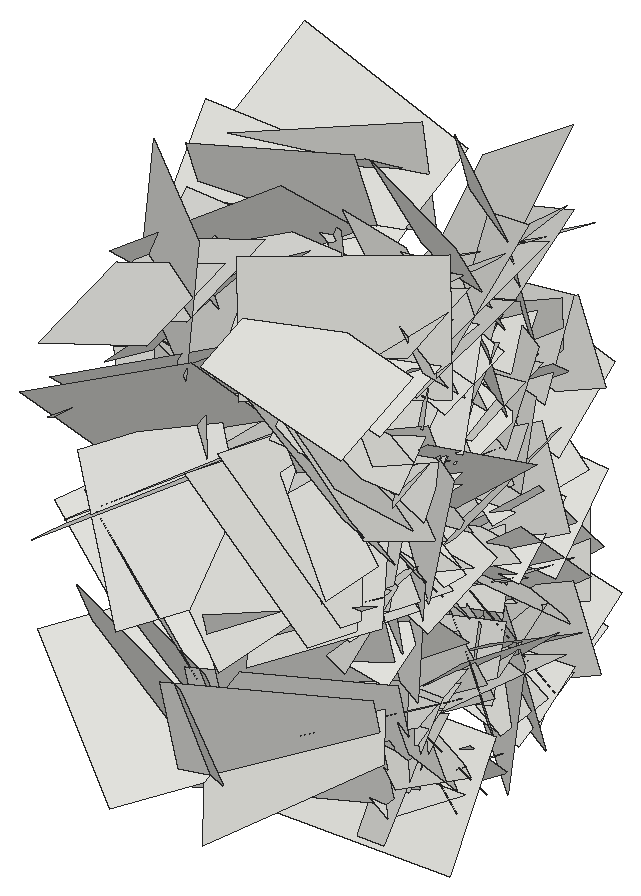
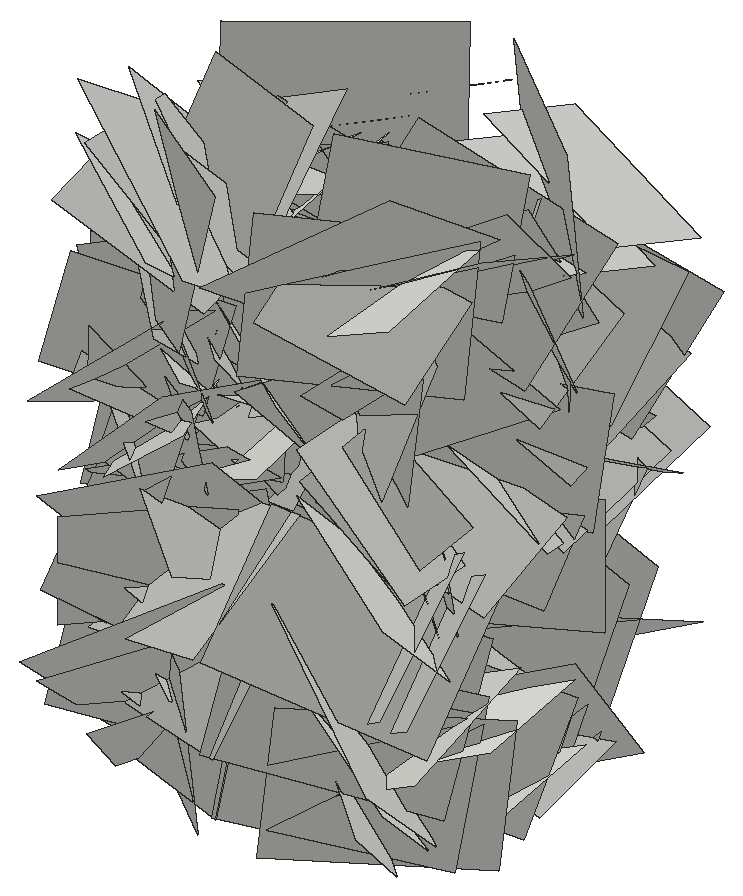
# SketchUp Ruby script. Lengths in inches.
U = 1.inch
M = Sketchup.active_model
def pt(a) = Geom::Point3d.new(a.map { |v| v * U })
def face(e, loops, mat)
  f = e.add_face(loops[0].map { |a| pt(a) })
  loops[1..].each { |l| e.add_face(l.map { |a| pt(a) }).erase! }
  f.material = f.back_material = mat if mat
  f
end
# faces: each face lists its corners as indices into pts; further lists are holes
def faces(e, pts, list, mat = nil) = list.each { |f| face(e, (f[0].is_a?(Array) ? f : [f]).map { |l| l.map { |i| pts[i] } }, mat) }
# xy, xz, yz: faces in a plane at the given z, y or x. An outline is a flat list of corners, or four numbers for a rectangle; further outlines are holes
def ring(l) = l.size == 4 ? [[l[0], l[1]], [l[2], l[1]], [l[2], l[3]], [l[0], l[3]]] : l.each_slice(2).to_a
def flat(e, list, mat, &to3) = list.each { |f| face(e, (f[0].is_a?(Array) ? f : [f]).map { |l| ring(l).map { |u, v| to3.(u, v) } }, mat) }
def xy(e, z, list, mat = nil) = flat(e, list, mat) { |x, y| [x, y, z] }
def xz(e, y, list, mat = nil) = flat(e, list, mat) { |x, z| [x, y, z] }
def yz(e, x, list, mat = nil) = flat(e, list, mat) { |y, z| [x, y, z] }
def lines(e, pts, list) = list.each { |a, b| e.add_line(pt(pts[a]), pt(pts[b])) }
# prism: a flat outline (further loops are holes) pulled along v
def prism(e, loops, v, mat = nil)
  f = face(e, loops, mat); d = Geom::Vector3d.new(v.map { |x| x * U })
  f.pushpull(f.normal.samedirection?(d) ? d.length : -d.length)
end
def box(e, o, s, mat = nil) = prism(e, [[o, [o[0] + s[0], o[1], o[2]], [o[0] + s[0], o[1] + s[1], o[2]], [o[0], o[1] + s[1], o[2]]]], [0, 0, s[2]], mat)
def at(x, y, z, deg = 0) = Geom::Transformation.translation(pt([x, y, z])) * Geom::Transformation.rotation(ORIGIN, Z_AXIS, deg.degrees)
def axes(o, x, y, z) = Geom::Transformation.new([*x, 0, *y, 0, *z, 0, *pt(o).to_a, 1])
def part(name) = M.definitions.add(name)
# library, detail: a bought-in or finely detailed component or shape, given as its bounding box
def library(name, o, s) = part(name).tap { |d| box(d.entities, o, s) }
def detail(e, o, s) = box(e.add_group.entities, o, s)
def put(e, d, t, mat = nil) = e.add_instance(d, t).tap { |i| i.material = mat if mat }
def group(e, t, mat = nil) = e.add_group.tap { |g| g.transformation = t; g.material = mat if mat }.entities
root = M.entities
c1 = part("Component\#6")
p = [[0.01,0,0],[0,3.24,4.54],[4.32,3.24,4.54],[4.33,0,0]]
faces(c1.entities,p,[[0,1,2,3]])
put(root,c1,axes([400.91,133.2,0.29],[-0.16868,0.00753,1.30134],[-0.16064,1.302,-0.02607],[1.37005,0.15359,0.15716]))
put(root,c1,axes([404.88,127.28,0.51],[0.04452,-0.40985,0.5808],[0.07759,0.58122,0.40485],[-0.7495,0.03582,0.07641]))
put(root,c1,axes([400.91,129.68,16.21],[0.16446,-0.17941,-0.82447],[0.07006,-0.83314,0.19373],[0.89165,0.09856,0.13685]))
put(root,c1,axes([404.88,134.26,15.51],[0.13639,0.72841,-0.25059],[0.07067,-0.26364,-0.7321],[-0.81346,0.09922,-0.10562]))
put(root,c1,axes([400.91,128.87,2.92],[0.01411,0.95221,-0.19006],[0.11482,-0.19035,-0.94606],[1.02282,0.00823,0.10882]))
put(root,c1,axes([400.91,138.97,11.375],[-0.02639,-0.72989,-0.72722],[0.07911,-0.7268,0.72691],[1.08928,0.0351,-0.07041]))
put(root,c1,axes([400.91,131.74,20.5625],[-0.11289,-0.41624,-1.03402],[0.06809,-1.03929,0.41174],[1.17957,0.02016,-0.12272]))
put(root,c1,axes([404.88,131.9,7.66],[0.03371,0.19161,0.61883],[0.06203,0.6162,-0.1938],[-0.68388,0.06533,0.01292]))
put(root,c1,axes([400.91,134.95,12.42],[0.03363,0.92541,-1.00089],[-0.39451,-0.95725,-0.89685],[1.39004,-0.29406,-0.23032]))
put(root,c1,axes([404.88,131.8,8.64],[0.08497,0.05507,0.67491],[0.04101,0.67814,-0.05993],[-0.71661,0.04534,0.0766]))
put(root,c1,axes([400.91,137.89,18.97],[0.02244,-0.79516,0.48934],[0.22215,0.48102,0.77258],[0.96443,-0.0923,-0.18934]))
put(root,c1,axes([400.91,137.87,11.82],[0.23548,-0.98581,-0.19043],[-0.17104,-0.22756,0.98976],[1.05044,0.18394,0.20385]))
put(root,c1,axes([400.91,129.625,19.87],[-0.14331,0.9196,0.97349],[-0.15794,0.96203,-0.92947],[1.41069,0.20113,-0.00516]))
put(root,c1,axes([400.91,130.99,8.6],[0.04494,-0.64922,0.68663],[0.20873,0.6783,0.62918],[0.97967,-0.11474,-0.16555]))
put(root,c1,axes([400.91,133.91,11.1875],[-0.02059,0.92356,-0.8814],[-0.20413,-0.87353,-0.91107],[1.33776,-0.11908,-0.15259]))
put(root,c1,axes([400.91,128.56,10.3125],[-0.23413,0.04823,1.24691],[0.1221,1.26168,-0.02839],[1.31707,-0.10839,0.22429]))
put(root,c1,axes([400.91,131.94,16.85],[-0.08825,-0.96476,0.81898],[-0.08011,0.82307,0.9619],[1.33903,-0.01434,0.11152]))
put(root,c1,axes([400.91,131.18,15.16],[0.15294,-1.16278,0.39158],[-0.28955,0.35393,1.15166],[1.26792,0.22109,0.21577]))
put(root,c1,axes([404.88,134.77,2.57],[0.05447,0.40704,0.46107],[0.08155,0.45478,-0.41007],[-0.64681,0.09162,-0.01288]))
put(root,c1,axes([400.91,134.14,22.88],[0.03825,0.99518,-0.25742],[0.13842,-0.25993,-0.98657],[1.08078,-0.00193,0.13547]))
put(root,c1,axes([400.19,124.93,11.12],[0.54058,0.75668,0.32998],[0.30141,0.20311,-0.90522],[0.82148,-0.57246,0.11499]))
put(root,c1,axes([400.91,127.92,6.47],[-0.03611,0.05394,1.13531],[0.09971,1.13206,-0.05096],[1.20066,-0.09239,0.03838]))
put(root,c1,axes([404.88,138.1,17.99],[0.00934,-0.49027,-0.41508],[0.1892,-0.3969,0.47259],[-0.65411,-0.1218,0.13076]))
put(root,c1,axes([400.91,127.69,20.12],[-0.02742,-1.01137,-0.35231],[0.21232,-0.35076,0.99222],[1.1152,0.04191,-0.19757]))
put(root,c1,axes([400.91,130,20.12],[-0.02742,-1.01137,-0.35231],[0.21232,-0.35076,0.99222],[1.1152,0.04191,-0.19757]))
put(root,c1,axes([404.88,129.35,18.22],[0.07955,-0.40219,0.442],[0.06566,0.44831,0.39741],[-0.63004,-0.00406,0.09723]))
put(root,c1,axes([400.91,129.81,24.32],[-0.08615,-0.07511,-1.33483],[-0.12267,-1.33188,0.08199],[1.41184,-0.12031,-0.07433]))
put(root,c1,axes([400.91,131.16,1.32],[0.11103,-1.00768,0.14491],[0.13016,0.15712,1.00381],[1.07125,0.08535,-0.13699]))
put(root,c1,axes([400.91,136.29,19.65],[0.239,0.33681,-1.04778],[-0.13934,-1.05364,-0.36698],[1.15826,-0.19625,0.17205]))
put(root,c1,axes([400.91,129.42,5.47],[-0.26825,1.30607,0.06413],[0.25565,0.11082,-1.30519],[1.36232,0.23638,0.25756]))
put(root,c1,axes([400.91,126.61,12.8],[-0.1414,-0.87971,0.87765],[0.19082,0.8597,0.88908],[1.30331,-0.22132,-0.03495]))
put(root,c1,axes([400.91,133.96,9.66],[0.06967,-1.04066,0.34132],[0.1454,0.34706,1.03175],[1.15177,0.01914,-0.15089]))
put(root,c1,axes([400.91,134.94,17.85],[0.08672,-0.29938,1.1859],[-0.04442,1.18717,0.30259],[1.29573,0.06074,-0.069]))
put(root,c1,axes([400.91,129.48,20.64],[-0.14207,1.22324,0.51937],[0.11373,0.53026,-1.2212],[1.40407,0.08082,0.15147]))
put(root,c1,axes([400.91,129.66,12.47],[-0.1081,-1.2535,0.58167],[-0.00417,0.58351,1.25678],[1.46479,-0.09085,0.0465]))
put(root,c1,axes([400.91,125.82,11.42],[0.20547,0.4933,-0.99975],[0.03886,-1.01702,-0.49472],[1.18108,-0.05236,0.1902]))
put(root,c1,axes([400.91,131.95,0.87],[0.07095,-0.70744,0.83659],[0.30432,0.82019,0.6706],[1.12076,-0.17792,-0.23504]))
put(root,c1,axes([400.91,139.8125,5.82],[0.12038,-0.94885,-0.86303],[-0.08352,-0.86993,0.94607],[1.35702,0.03063,0.13479]))
put(root,c1,axes([400.91,133.04,19.75],[0.14526,-0.49923,0.95494],[0.24012,0.95446,0.46647],[1.11669,-0.1403,-0.22453]))
put(root,c1,axes([400.91,128.24,17.68],[0.22785,0.52614,1.07761],[-0.06777,1.09826,-0.52347],[1.26934,-0.03581,-0.22138]))
put(root,c1,axes([400.91,133.15,22.79],[0.15509,1.06813,0.73269],[-0.10614,0.74447,-1.06531],[1.36888,-0.06329,-0.16562]))
put(root,c1,axes([400.91,132.12,7.08],[-0.00585,1.22451,-0.43101],[0.11167,-0.42917,-1.22063],[1.3715,0.04016,0.09755]))
put(root,c1,axes([400.91,125.99,1.35],[0.00241,0.79041,1.08039],[0.06651,1.07914,-0.78963],[1.41741,-0.05198,0.03522]))
put(root,c1,axes([400.91,127.67,13.74],[0.06329,-0.97705,0.81505],[0.12838,0.8166,0.97005],[1.34259,-0.03203,-0.13118]))
put(root,c1,axes([400.91,137,19.49],[0.23927,-0.1296,-1.18474],[0.04055,-1.20439,0.13904],[1.26266,0.06324,0.22004]))
put(root,c1,axes([400.91,135.39,1.18],[0.01455,-0.40823,1.27358],[0.1801,1.26386,0.40328],[1.40617,-0.15765,-0.06483]))
put(root,c1,axes([400.91,128.0625,10.23],[0.10909,-1.3698,0.20566],[-0.00727,0.20572,1.37363],[1.46824,0.1028,-0.00848]))
put(root,c1,axes([400.91,129.98,10.23],[0.10909,-1.3698,0.20566],[-0.00727,0.20572,1.37363],[1.46824,0.1028,-0.00848]))
put(root,c1,axes([400.91,138.98,4.78],[0.22268,-0.9196,-0.8307],[0.07298,-0.83259,0.9391],[1.31157,0.20246,0.08879]))
put(root,c1,axes([399.74,124.5,5.79],[0.83668,1.07369,0.2523],[0.21003,0.16716,-1.33127],[1.15009,-0.81162,0.05958]))
put(root,c1,axes([400.91,130.78,10.54],[0.24762,-1.26357,-0.1726],[-0.00687,-0.17664,1.28442],[1.3518,0.23056,0.03815]))
put(root,c1,axes([400.91,136.82,5.83],[0.1656,-1.02965,0.80161],[0.14776,0.81588,1.02082],[1.37528,0.03632,-0.2062]))
put(root,c1,axes([400.91,130.15,15.41],[0.24379,0.89731,1.03665],[0.02149,1.04879,-0.91232],[1.45316,-0.16605,-0.16042]))
put(root,c1,axes([400.91,135.96,3.29],[0.1622,-0.76384,1.11136],[0.23079,1.11781,0.7383],[1.4107,-0.09505,-0.24857]))
put(root,c1,axes([400.91,125.3125,7.6875],[0.15543,0.49215,-1.26812],[0.29157,-1.25984,-0.45713],[1.41209,0.20597,0.23397]))
put(root,c1,axes([400.91,126.76,7.6875],[0.15543,0.49215,-1.26812],[0.29157,-1.25984,-0.45713],[1.41209,0.20597,0.23397]))
put(root,c1,axes([400.8,125.5,13.2],[1.07209,0.56535,0.5401],[0.40295,0.41611,-1.14744],[0.72423,-1.06841,-0.1611]))
put(root,c1,axes([414.79,125.5,13.2],[-1.07209,0.56535,0.5401],[-0.40295,0.41611,-1.14744],[-0.72423,-1.06841,-0.1611]))
put(root,c1,axes([414.68,125.3125,7.6875],[-0.15543,0.49215,-1.26812],[-0.29157,-1.25984,-0.45713],[-1.41209,0.20597,0.23397]))
put(root,c1,axes([414.68,126.76,7.6875],[-0.15543,0.49215,-1.26812],[-0.29157,-1.25984,-0.45713],[-1.41209,0.20597,0.23397]))
put(root,c1,axes([414.68,135.96,3.29],[-0.1622,-0.76384,1.11136],[-0.23079,1.11781,0.7383],[-1.4107,-0.09505,-0.24857]))
put(root,c1,axes([414.68,130.15,15.41],[-0.24379,0.89731,1.03665],[-0.02149,1.04879,-0.91232],[-1.45316,-0.16605,-0.16042]))
put(root,c1,axes([414.68,136.82,5.83],[-0.1656,-1.02965,0.80161],[-0.14776,0.81588,1.02082],[-1.37528,0.03632,-0.2062]))
put(root,c1,axes([414.68,130.78,10.54],[-0.24762,-1.26357,-0.1726],[0.00687,-0.17664,1.28442],[-1.3518,0.23056,0.03815]))
put(root,c1,axes([415.85,124.5,5.79],[-0.83668,1.07369,0.2523],[-0.21003,0.16716,-1.33127],[-1.15009,-0.81162,0.05958]))
put(root,c1,axes([414.68,138.98,4.78],[-0.22268,-0.9196,-0.8307],[-0.07298,-0.83259,0.9391],[-1.31157,0.20246,0.08879]))
put(root,c1,axes([414.68,128.0625,10.23],[-0.10909,-1.3698,0.20566],[0.00727,0.20572,1.37363],[-1.46824,0.1028,-0.00848]))
put(root,c1,axes([414.68,129.98,10.23],[-0.10909,-1.3698,0.20566],[0.00727,0.20572,1.37363],[-1.46824,0.1028,-0.00848]))
put(root,c1,axes([414.68,135.39,1.18],[-0.01455,-0.40823,1.27358],[-0.1801,1.26386,0.40328],[-1.40617,-0.15765,-0.06483]))
put(root,c1,axes([414.68,137,19.49],[-0.23927,-0.1296,-1.18474],[-0.04055,-1.20439,0.13904],[-1.26266,0.06324,0.22004]))
put(root,c1,axes([414.68,127.67,13.74],[-0.06329,-0.97705,0.81505],[-0.12838,0.8166,0.97005],[-1.34259,-0.03203,-0.13118]))
put(root,c1,axes([414.68,125.99,1.35],[-0.00241,0.79041,1.08039],[-0.06651,1.07914,-0.78963],[-1.41741,-0.05198,0.03522]))
put(root,c1,axes([414.68,132.12,7.08],[0.00585,1.22451,-0.43101],[-0.11167,-0.42917,-1.22063],[-1.3715,0.04016,0.09755]))
put(root,c1,axes([414.68,133.15,22.79],[-0.15509,1.06813,0.73269],[0.10614,0.74447,-1.06531],[-1.36888,-0.06329,-0.16562]))
put(root,c1,axes([414.68,128.24,17.68],[-0.22785,0.52614,1.07761],[0.06777,1.09826,-0.52347],[-1.26934,-0.03581,-0.22138]))
put(root,c1,axes([414.68,133.04,19.75],[-0.14526,-0.49923,0.95494],[-0.24012,0.95446,0.46647],[-1.11669,-0.1403,-0.22453]))
put(root,c1,axes([414.68,139.8125,5.82],[-0.12038,-0.94885,-0.86303],[0.08352,-0.86993,0.94607],[-1.35702,0.03063,0.13479]))
put(root,c1,axes([414.68,131.95,0.87],[-0.07095,-0.70744,0.83659],[-0.30432,0.82019,0.6706],[-1.12076,-0.17792,-0.23504]))
put(root,c1,axes([414.68,125.82,11.42],[-0.20547,0.4933,-0.99975],[-0.03886,-1.01702,-0.49472],[-1.18108,-0.05236,0.1902]))
put(root,c1,axes([414.68,129.66,12.47],[0.1081,-1.2535,0.58167],[0.00417,0.58351,1.25678],[-1.46479,-0.09085,0.0465]))
put(root,c1,axes([414.68,129.48,20.64],[0.14207,1.22324,0.51937],[-0.11373,0.53026,-1.2212],[-1.40407,0.08082,0.15147]))
put(root,c1,axes([414.68,134.94,17.85],[-0.08672,-0.29938,1.1859],[0.04442,1.18717,0.30259],[-1.29573,0.06074,-0.069]))
put(root,c1,axes([414.68,133.96,9.66],[-0.06967,-1.04066,0.34132],[-0.1454,0.34706,1.03175],[-1.15177,0.01914,-0.15089]))
put(root,c1,axes([414.68,126.61,12.8],[0.1414,-0.87971,0.87765],[-0.19082,0.8597,0.88908],[-1.30331,-0.22132,-0.03495]))
put(root,c1,axes([414.68,129.42,5.47],[0.26825,1.30607,0.06413],[-0.25565,0.11082,-1.30519],[-1.36232,0.23638,0.25756]))
put(root,c1,axes([414.68,136.29,19.65],[-0.239,0.33681,-1.04778],[0.13934,-1.05364,-0.36698],[-1.15826,-0.19625,0.17205]))
put(root,c1,axes([414.68,131.16,1.32],[-0.11103,-1.00768,0.14491],[-0.13016,0.15712,1.00381],[-1.07125,0.08535,-0.13699]))
put(root,c1,axes([414.68,129.81,24.32],[0.08615,-0.07511,-1.33483],[0.12267,-1.33188,0.08199],[-1.41184,-0.12031,-0.07433]))
put(root,c1,axes([410.71,129.35,18.22],[-0.07955,-0.40219,0.442],[-0.06566,0.44831,0.39741],[0.63004,-0.00406,0.09723]))
put(root,c1,axes([414.68,127.69,20.12],[0.02742,-1.01137,-0.35231],[-0.21232,-0.35076,0.99222],[-1.1152,0.04191,-0.19757]))
put(root,c1,axes([414.68,130,20.12],[0.02742,-1.01137,-0.35231],[-0.21232,-0.35076,0.99222],[-1.1152,0.04191,-0.19757]))
put(root,c1,axes([410.71,138.1,17.99],[-0.00934,-0.49027,-0.41508],[-0.1892,-0.3969,0.47259],[0.65411,-0.1218,0.13076]))
put(root,c1,axes([414.68,127.92,6.47],[0.03611,0.05394,1.13531],[-0.09971,1.13206,-0.05096],[-1.20066,-0.09239,0.03838]))
put(root,c1,axes([415.4,124.93,11.12],[-0.54058,0.75668,0.32998],[-0.30141,0.20311,-0.90522],[-0.82148,-0.57246,0.11499]))
put(root,c1,axes([414.68,134.14,22.88],[-0.03825,0.99518,-0.25742],[-0.13842,-0.25993,-0.98657],[-1.08078,-0.00193,0.13547]))
put(root,c1,axes([410.71,134.77,2.57],[-0.05447,0.40704,0.46107],[-0.08155,0.45478,-0.41007],[0.64681,0.09162,-0.01288]))
put(root,c1,axes([414.68,131.18,15.16],[-0.15294,-1.16278,0.39158],[0.28955,0.35393,1.15166],[-1.26792,0.22109,0.21577]))
put(root,c1,axes([414.68,131.94,16.85],[0.08825,-0.96476,0.81898],[0.08011,0.82307,0.9619],[-1.33903,-0.01434,0.11152]))
put(root,c1,axes([414.68,128.56,10.3125],[0.23413,0.04823,1.24691],[-0.1221,1.26168,-0.02839],[-1.31707,-0.10839,0.22429]))
put(root,c1,axes([414.68,133.91,11.1875],[0.02059,0.92356,-0.8814],[0.20413,-0.87353,-0.91107],[-1.33776,-0.11908,-0.15259]))
put(root,c1,axes([414.68,130.99,8.6],[-0.04494,-0.64922,0.68663],[-0.20873,0.6783,0.62918],[-0.97967,-0.11474,-0.16555]))
put(root,c1,axes([414.68,129.625,19.87],[0.14331,0.9196,0.97349],[0.15794,0.96203,-0.92947],[-1.41069,0.20113,-0.00516]))
put(root,c1,axes([414.68,137.87,11.82],[-0.23548,-0.98581,-0.19043],[0.17104,-0.22756,0.98976],[-1.05044,0.18394,0.20385]))
put(root,c1,axes([410.71,131.8,8.64],[-0.08497,0.05507,0.67491],[-0.04101,0.67814,-0.05993],[0.71661,0.04534,0.0766]))
put(root,c1,axes([414.68,134.95,12.42],[-0.03363,0.92541,-1.00089],[0.39451,-0.95725,-0.89685],[-1.39004,-0.29406,-0.23032]))
put(root,c1,axes([410.71,131.9,7.66],[-0.03371,0.19161,0.61883],[-0.06203,0.6162,-0.1938],[0.68388,0.06533,0.01292]))
put(root,c1,axes([414.68,131.74,20.5625],[0.11289,-0.41624,-1.03402],[-0.06809,-1.03929,0.41174],[-1.17957,0.02016,-0.12272]))
put(root,c1,axes([414.68,138.97,11.375],[0.02639,-0.72989,-0.72722],[-0.07911,-0.7268,0.72691],[-1.08928,0.0351,-0.07041]))
put(root,c1,axes([414.68,128.87,2.92],[-0.01411,0.95221,-0.19006],[-0.11482,-0.19035,-0.94606],[-1.02282,0.00823,0.10882]))
put(root,c1,axes([410.71,134.26,15.51],[-0.13639,0.72841,-0.25059],[-0.07067,-0.26364,-0.7321],[0.81346,0.09922,-0.10562]))
put(root,c1,axes([414.68,129.68,16.21],[-0.16446,-0.17941,-0.82447],[-0.07006,-0.83314,0.19373],[-0.89165,0.09856,0.13685]))
put(root,c1,axes([410.71,127.28,0.51],[-0.04452,-0.40985,0.5808],[-0.07759,0.58122,0.40485],[0.7495,0.03582,0.07641]))
put(root,c1,axes([414.68,133.2,0.29],[0.16868,0.00753,1.30134],[0.16064,1.302,-0.02607],[-1.37005,0.15359,0.15716]))
put(root,c1,axes([410.71,134.57,7.51],[-0.06425,-0.0713,-0.65597],[0.02618,-0.65852,0.06929],[0.69893,0.01811,-0.0629]))
put(root,c1,axes([414.68,128.52,17.74],[-0.08604,0.43028,-0.81229],[-0.04293,-0.81633,-0.42838],[-0.97342,-0.00203,0.0907]))
put(root,c1,axes([410.71,132.11,13.83],[-0.12823,-0.67114,-0.46171],[-0.10246,-0.45164,0.68184],[0.85739,-0.15435,0.01243]))
put(root,c1,axes([414.68,133.79,15.82],[-0.11741,-0.82822,-0.37202],[-0.00882,-0.37384,0.83474],[-0.96237,0.10447,0.03774]))
put(root,c1,axes([410.71,131.53,3.64],[-0.03356,0.34972,-0.55611],[0.01458,-0.55628,-0.35061],[0.69619,0.02851,-0.01946]))
put(root,c1,axes([410.71,130.57,14.69],[-0.08088,0.56373,-0.36339],[0.06437,-0.35843,-0.56878],[0.70803,0.09698,0.0102]))
put(root,c1,axes([414.68,130.125,12.36],[0.14413,1.23778,0.56401],[0.30073,0.52855,-1.22835],[-1.41013,0.23923,-0.20431]))
put(root,c1,axes([414.68,129.28,18.375],[-0.15104,-0.37703,-0.77667],[0.00911,-0.78776,0.38083],[-0.9151,0.05438,0.13199]))
put(root,c1,axes([414.68,132.6,22.9],[-0.05818,0.99288,0.05669],[0.07779,0.06066,-0.99145],[-1.05129,-0.05046,-0.07649]))
put(root,c1,axes([410.71,133.3125,17.59],[0.01529,0.27468,0.5349],[0.08187,0.52978,-0.27413],[0.6321,-0.07526,0.02257]))
put(root,c1,axes([410.71,129.84,16.13],[0.05288,0.68465,0.04631],[-0.09068,0.05228,-0.68068],[0.72171,-0.04359,-0.08892]))
put(root,c1,axes([414.68,129.45,15.69],[0.00555,0.72683,0.86308],[0.19522,0.85097,-0.71774],[-1.18002,0.1442,-0.11468]))
put(root,c1,axes([410.71,129.41,10.95],[-0.18775,-0.48629,-0.69123],[0.00245,-0.70652,0.49646],[0.89586,-0.09998,-0.14623]))
put(root,c1,axes([410.71,132.63,6.14],[-0.10731,0.87556,-0.00554],[-0.12201,-0.01884,-0.87366],[0.92006,0.09962,-0.1165]))
put(root,c1,axes([414.68,133.96,12.5],[-0.03937,0.24323,0.81298],[-0.12274,0.80469,-0.24604],[-0.89109,-0.12158,-0.00203]))
put(root,c1,axes([414.68,127.6,6.32],[-0.09105,0.77875,-0.27248],[-0.08108,-0.28029,-0.77696],[-0.87078,-0.05533,0.10084]))
put(root,c1,axes([414.68,133.1,9.3125],[0.02086,0.87239,-0.16813],[-0.14049,-0.16341,-0.8634],[-0.93122,0.04419,0.12649]))
put(root,c1,axes([414.68,131.05,1.96],[0.03915,-1.05631,0.36623],[0.17317,0.36759,1.04378],[-1.17236,0.01903,0.16641]))
put(root,c1,axes([410.71,133.88,6.93],[-0.12434,-0.60409,0.41763],[0.12699,0.40152,0.61444],[0.76804,-0.16419,-0.03398]))
put(root,c1,axes([414.68,136.93,7.59],[0.11136,0.24127,-0.97313],[-0.07388,-0.97433,-0.24909],[-1.06018,0.09324,-0.08486]))
put(root,c1,axes([410.71,130.03,2.94],[-0.11679,-0.3481,0.76621],[-0.04914,0.77408,0.34502],[0.89071,-0.00294,0.1195]))
put(root,c1,axes([410.71,129.23,5.41],[-0.17398,-0.60139,0.60701],[0.02487,0.6147,0.61536],[0.9054,-0.13245,0.09973]))
put(root,c1,axes([414.68,132.5,3.06],[0.12033,-0.77552,-0.96336],[0.26418,-0.93322,0.78062],[-1.28404,-0.26468,0.07033]))
put(root,c1,axes([410.71,129.18,10.77],[0.08644,0.04023,-0.60323],[0.06997,-0.60565,-0.03147],[0.63702,0.06107,0.08531]))
put(root,c1,axes([414.68,132.55,10.48],[0.11298,-1.07137,-0.22101],[0.09706,-0.21254,1.07447],[-1.1555,-0.12261,0.06864]))
put(root,c1,axes([410.71,128.34,18.92],[0.04874,0.38349,0.62334],[-0.06251,0.62448,-0.37984],[0.77325,0.02631,-0.07]))
put(root,c1,axes([410.71,129.8,15.91],[0.05085,-0.71724,0.33006],[-0.13843,0.31891,0.71198],[0.82538,0.09767,0.09907]))
put(root,c1,axes([414.68,127.86,19.19],[0.25173,1.01088,0.57921],[0.04385,0.58343,-1.03521],[-1.23418,0.22691,0.08136]))
put(root,c1,axes([414.68,127.34,21.1],[0.03089,0.79811,0.32897],[-0.11706,0.3299,-0.79059],[-0.90753,-0.01539,0.11317]))
put(root,c1,axes([410.71,133.42,16.97],[-0.14677,0.94615,0.46149],[-0.22557,0.4307,-0.94687],[1.09283,0.21597,-0.13346]))
put(root,c1,axes([410.71,133.96,6.46],[-0.0893,0.11056,0.97068],[-0.19494,0.95507,-0.12474],[1.01706,0.19277,0.06132]))
put(root,c1,axes([414.68,136.53,11.26],[0.01536,-0.64622,-0.54667],[-0.11065,-0.54394,0.64022],[-0.89037,0.05645,-0.089]))
put(root,c1,axes([410.71,131.99,-0.9375],[0.0225,-0.54484,0.50649],[-0.02225,0.50605,0.54525],[0.78821,0.02984,0.00093]))
put(root,c1,axes([414.68,127.95,5.4],[-0.05879,0.74539,0.22064],[-0.10629,0.21249,-0.74307],[-0.81711,-0.08127,0.08079]))
put(root,c1,axes([410.71,125.86,8.82],[0.02658,0.53015,0.39509],[0.11889,0.38623,-0.52538],[0.69069,-0.08688,0.07523]))
put(root,c1,axes([410.71,131.86,3.01],[0.01467,-0.55248,-0.51034],[-0.00827,-0.51051,0.55244],[0.7972,0.00487,0.01512]))
put(root,c1,axes([410.71,136.82,15.87],[-0.16772,-0.74319,-0.48228],[0.03783,-0.49486,0.75087],[0.93836,-0.11289,-0.11647]))
put(root,c1,axes([414.68,125.93,11.7],[-0.16945,0.67455,-0.05214],[-0.09647,-0.07453,-0.68517],[-0.71064,-0.15073,0.10544]))
put(root,c1,axes([414.68,127.92,4.7],[-0.092,0.70183,0.2556],[-0.07294,0.24871,-0.70628],[-0.78837,-0.10491,0.03552]))
put(root,c1,axes([414.68,128.53,16.93],[0.30517,1.08519,-0.55956],[0.1011,-0.59314,-1.10124],[-1.29027,0.21019,-0.21864]))
put(root,c1,axes([410.71,137.37,4.77],[-0.01509,-0.67708,-0.46908],[-0.05072,-0.46768,0.67651],[0.87164,-0.03894,0.03124]))
put(root,c1,axes([414.68,133.14,16.06],[0.03738,-0.31853,0.81486],[-0.04959,0.81367,0.32009],[-0.92608,-0.05642,0.01575]))
put(root,c1,axes([414.68,133.58,20.74],[0.06025,0.71815,0.57437],[0.00066,0.57544,-0.71955],[-0.97476,0.04478,0.03501]))
put(root,c1,axes([414.68,131.35,15.19],[-0.02447,0.82058,-0.14823],[-0.01236,-0.14859,-0.82075],[-0.8838,-0.02064,0.01558]))
put(root,c1,axes([410.71,130.01,4.69],[0.05447,0.12092,0.77662],[-0.06993,0.77619,-0.11649],[0.83019,0.05744,-0.06077]))
put(root,c1,axes([414.68,135.14,15.06],[0.15738,0.18416,-1.10832],[0.16264,-1.1108,-0.16402],[-1.17977,-0.12857,-0.17046]))
put(root,c1,axes([414.68,133.07,14.74],[0.12706,0.28525,0.91315],[-0.02767,0.92092,-0.28425],[-1.01369,0.01061,0.12222]))
put(root,c1,axes([414.68,132.96,18.89],[0.10145,-0.91774,-0.17179],[-0.02227,-0.17476,0.92192],[-0.98945,-0.09016,-0.03837]))
put(root,c1,axes([410.71,135.65,2.32],[-0.1935,-1.06071,0.09437],[-0.13048,0.11613,1.0671],[1.12123,-0.16954,0.14047]))
put(root,c1,axes([410.71,136.42,13.64],[0.14309,-0.55174,0.41683],[-0.03038,0.41987,0.56505],[0.73236,0.12522,-0.058]))
put(root,c1,axes([414.68,137.27,19.36],[0.1763,0.15017,-0.9005],[-0.15684,-0.89878,-0.17721],[-0.95491,0.17535,-0.13715]))
put(root,c1,axes([414.68,130.2,1.79],[0.1042,-0.77086,0.73803],[0.17604,0.74317,0.75412],[-1.11745,0.04519,0.18762]))
put(root,c1,axes([414.68,136.01,11.51],[-0.06598,-0.27091,0.62957],[-0.16839,0.62065,0.25136],[-0.70672,-0.12259,-0.11867]))
put(root,c1,axes([410.71,133.51,8.98],[-0.15319,0.47062,-0.90401],[-0.09722,-0.91536,-0.46187],[1.07594,-0.0157,-0.17044]))
put(root,c1,axes([414.68,126.24,11.02],[-0.17433,0.41563,0.4957],[-0.04437,0.50356,-0.43611],[-0.68427,-0.13854,-0.09801]))
